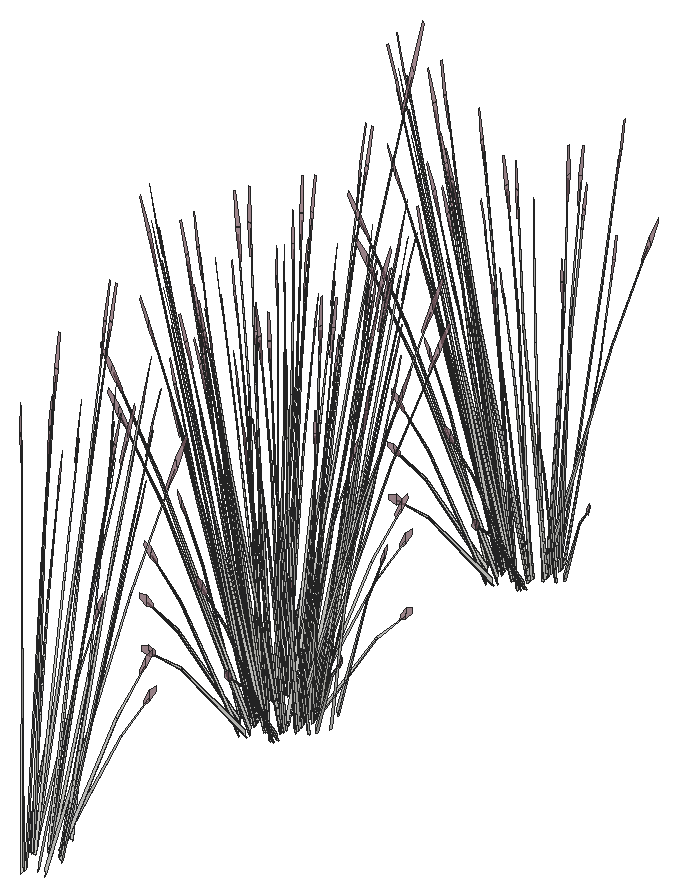
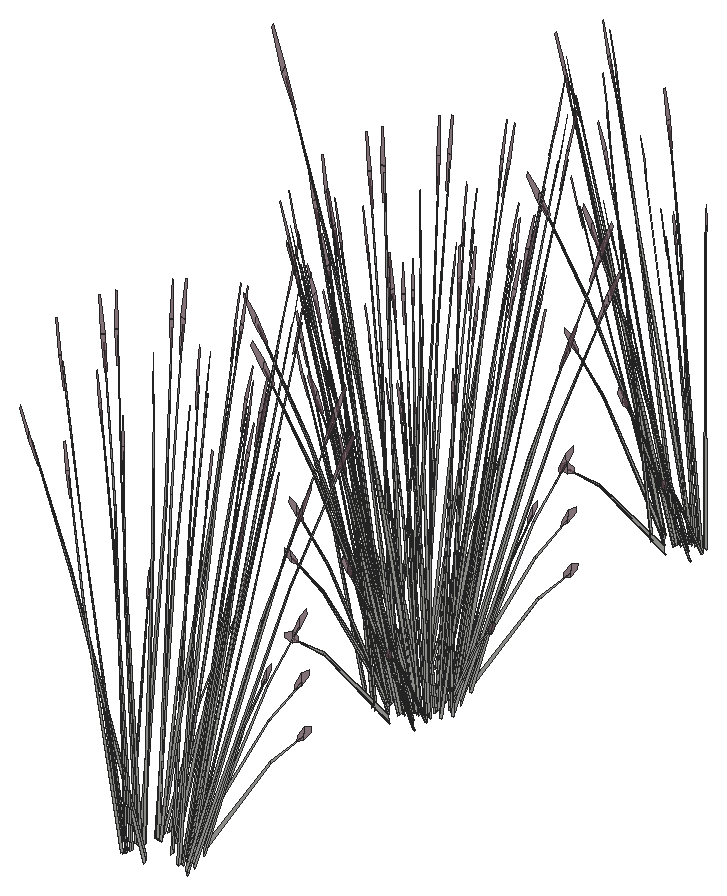
# SketchUp Ruby script. Lengths in inches.
U = 1.inch
M = Sketchup.active_model
def pt(a) = Geom::Point3d.new(a.map { |v| v * U })
def face(e, loops, mat)
  f = e.add_face(loops[0].map { |a| pt(a) })
  loops[1..].each { |l| e.add_face(l.map { |a| pt(a) }).erase! }
  f.material = f.back_material = mat if mat
  f
end
# faces: each face lists its corners as indices into pts; further lists are holes
def faces(e, pts, list, mat = nil) = list.each { |f| face(e, (f[0].is_a?(Array) ? f : [f]).map { |l| l.map { |i| pts[i] } }, mat) }
# xy, xz, yz: faces in a plane at the given z, y or x. An outline is a flat list of corners, or four numbers for a rectangle; further outlines are holes
def ring(l) = l.size == 4 ? [[l[0], l[1]], [l[2], l[1]], [l[2], l[3]], [l[0], l[3]]] : l.each_slice(2).to_a
def flat(e, list, mat, &to3) = list.each { |f| face(e, (f[0].is_a?(Array) ? f : [f]).map { |l| ring(l).map { |u, v| to3.(u, v) } }, mat) }
def xy(e, z, list, mat = nil) = flat(e, list, mat) { |x, y| [x, y, z] }
def xz(e, y, list, mat = nil) = flat(e, list, mat) { |x, z| [x, y, z] }
def yz(e, x, list, mat = nil) = flat(e, list, mat) { |y, z| [x, y, z] }
def lines(e, pts, list) = list.each { |a, b| e.add_line(pt(pts[a]), pt(pts[b])) }
# prism: a flat outline (further loops are holes) pulled along v
def prism(e, loops, v, mat = nil)
  f = face(e, loops, mat); d = Geom::Vector3d.new(v.map { |x| x * U })
  f.pushpull(f.normal.samedirection?(d) ? d.length : -d.length)
end
def box(e, o, s, mat = nil) = prism(e, [[o, [o[0] + s[0], o[1], o[2]], [o[0] + s[0], o[1] + s[1], o[2]], [o[0], o[1] + s[1], o[2]]]], [0, 0, s[2]], mat)
def at(x, y, z, deg = 0) = Geom::Transformation.translation(pt([x, y, z])) * Geom::Transformation.rotation(ORIGIN, Z_AXIS, deg.degrees)
def axes(o, x, y, z) = Geom::Transformation.new([*x, 0, *y, 0, *z, 0, *pt(o).to_a, 1])
def part(name) = M.definitions.add(name)
# library, detail: a bought-in or finely detailed component or shape, given as its bounding box
def library(name, o, s) = part(name).tap { |d| box(d.entities, o, s) }
def detail(e, o, s) = box(e.add_group.entities, o, s)
def put(e, d, t, mat = nil) = e.add_instance(d, t).tap { |i| i.material = mat if mat }
def group(e, t, mat = nil) = e.add_group.tap { |g| g.transformation = t; g.material = mat if mat }.entities
root = M.entities
M.materials.add("LightPink_Translucent").color = [144, 107, 117]
M.materials["LightPink_Translucent"].alpha = 0.75
c1 = part("blade")
p = [[2.15,0.21,22],[0,0.17,0],[0.09,0.45,0],[2.18,0.31,22],[2.29,0.31,22],[0.38,0.45,0],
  [2.48,0.24,33],[2.49,0.24,33],[2.48,0.22,33]]
faces(c1.entities,p,[[0,1,2,3],[4,5,2,3],[6,3,4,7],[8,0,3,6]])
c2 = part("seeds")
p = [[0.3,-0.1,1.38],[-0.01,-0.03,1.59],[-0.01,-0.03,0.03],[0.14,-0.07,-0.07],[0.29,-0.03,3],[0.15,0.01,3.11]]
faces(c2.entities,p,[[0,1,2,3],[1,0,4,5]],"LightPink_Translucent")
c3 = part("blade with seeds")
put(c3.entities,c1,at(0,0,0))
put(c3.entities,c2,axes([2.4,0.25,30.99],[1.5799,-0.05474,1.17369],[-0.12525,1.92788,0.29478],[-0.07173,-0.02425,1.56792]))
put(root,c3,axes([432.97,46.57,2.33],[0.22423,-0.47232,-0.10458],[0.32472,0.27211,-0.58045],[0.11288,0.13344,0.88199]))
put(root,c3,axes([431.35,44.86,1.33],[0.09398,-0.16955,1.47384],[0.23731,0.45764,0.11917],[-0.16276,0.20841,0.63005]))
put(root,c3,axes([431.49,45.93,2.34],[0.2546,-0.29052,0.30456],[0.24101,0.33173,-0.39319],[-0.03667,0.16855,0.75234]))
put(root,c3,axes([432.68,46.96,2.05],[0.00111,-0.06681,1.5255],[0.32247,-0.29474,-0.14414],[0.11201,0.1052,0.26996]))
put(root,c3,axes([431.26,46.2,2.07],[-0.30922,-0.02571,0.0553],[0.00848,-0.38824,0.43534],[-0.03236,0.14872,0.66383]))
put(root,c3,axes([431.36,46.23,2.07],[-0.26795,-0.37649,0.41282],[0.28456,-0.3247,0.34039],[-0.04943,0.17664,0.85423]))
put(root,c3,axes([432.21,46.41,2.34],[0.11344,-0.42434,0.30456],[0.33096,0.12377,-0.39319],[0.03035,0.17085,0.75234]))
put(root,c3,axes([433.05,46.74,2.07],[-0.17102,0.35053,0.0553],[-0.24354,-0.20408,0.43534],[0.07874,0.11238,0.66383]))
put(root,c3,axes([432.65,47.93,2.86],[0.26003,-0.31656,-0.05579],[0.23826,0.3467,-0.25298],[0.01677,0.09824,0.83441]))
put(root,c3,axes([433.125,46.65,2.07],[-0.37426,0.12663,0.41282],[-0.06495,-0.49674,0.34039],[0.08802,0.1464,0.85423]))
put(root,c3,axes([431.28,45.28,1.33],[0.07006,-0.18966,1.47384],[0.29392,0.3925,0.11917],[-0.13259,0.24463,0.63005]))
put(root,c3,axes([432.1,46.8,2.07],[-0.27727,0.18753,0.0553],[-0.13571,-0.34197,0.43534],[0.02678,0.15075,0.66383]))
put(root,c3,axes([430.48,46.26,2.05],[-0.00935,0.1092,1.50452],[0.26544,0.37987,-0.23794],[-0.06949,0.17964,0.12066]))
put(root,c3,axes([431.33,46.01,2.64],[0.41355,0.02734,-0.11608],[-0.0113,0.51765,-0.6443],[-0.02873,0.19937,0.97901]))
put(root,c3,axes([432.09,46.59,2.33],[0.36822,-0.25691,-0.10458],[0.18095,0.45596,-0.58045],[0.04858,0.19215,0.88199]))
put(root,c3,axes([432.2,46.76,2.35],[-0.37078,-0.14426,0.45823],[0.12679,-0.47426,0.37783],[0.02228,0.18651,0.9482]))
put(root,c3,axes([432.62,45.59,1.33],[-0.08601,-0.17716,1.47384],[0.39746,-0.14915,0.11917],[0.08983,0.27813,0.63005]))
put(root,c3,axes([430.45,47.38,2.05],[0.04269,-0.03331,1.5255],[0.35284,0.2216,-0.14414],[-0.00829,0.1845,0.26996]))
put(root,c3,axes([431.92,45.68,1.33],[-0.00921,-0.21179,1.47384],[0.39917,0.1405,0.11917],[-0.02469,0.30182,0.63005]))
put(root,c3,axes([432.01,47.61,2.05],[0.0477,0.08886,1.50452],[0.38493,0.03491,-0.23794],[0.03871,0.19596,0.12066]))
put(root,c3,axes([431.68,66.12,1.33],[0.08601,0.17716,1.47384],[-0.39746,0.14915,0.11917],[-0.08983,-0.27813,0.63005]))
put(root,c3,axes([432.33,64.95,2.05],[-0.05755,-0.07737,1.50452],[-0.38409,0.04905,-0.23794],[-0.0613,-0.18505,0.12066]))
put(root,c3,axes([434.06,65.89,2.05],[-0.00363,-0.10982,1.50452],[-0.30678,-0.3174,-0.23794],[0.04743,-0.1924,0.12066]))
put(root,c3,axes([433.02,66.43,1.33],[-0.07006,0.18966,1.47384],[-0.29392,-0.3925,0.11917],[0.13259,-0.24463,0.63005]))
put(root,c3,axes([433.98,65.5,2.05],[-0.03821,0.04215,1.5255],[-0.37441,-0.1422,-0.14414],[-0.01355,-0.18393,0.26996]))
put(root,c3,axes([431.9375,64.69,2.05],[-0.00702,0.06614,1.5255],[-0.34622,0.24004,-0.14414],[-0.10188,-0.1227,0.26996]))
put(root,c3,axes([431.86,65.87,2.38],[0.41917,-0.14183,0.46236],[0.07275,0.55635,0.38124],[-0.09858,-0.16397,0.95674]))
put(root,c3,axes([432.81,65.97,2.07],[0.37078,0.14426,0.41282],[-0.12679,0.47426,0.34039],[-0.02228,-0.18651,0.85423]))
put(root,c3,axes([432.92,66.14,2.33],[-0.36822,0.25691,-0.10458],[-0.18095,-0.45596,-0.58045],[-0.04858,-0.19215,0.88199]))
put(root,c3,axes([433.68,66.72,2.33],[-0.41355,-0.02734,-0.10458],[0.0113,-0.51765,-0.58045],[0.02873,-0.19937,0.88199]))
put(root,c3,axes([432.91,65.93,2.07],[0.27727,-0.18753,0.0553],[0.13571,0.34197,0.43534],[-0.02678,-0.15075,0.66383]))
put(root,c3,axes([431.96,65.99,2.07],[0.17102,-0.35053,0.0553],[0.24354,0.20408,0.43534],[-0.07874,-0.11238,0.66383]))
put(root,c3,axes([431.1,66.67,1.33],[0.13977,0.09507,1.47384],[-0.28925,0.39884,0.11917],[-0.18028,-0.17992,0.63005]))
put(root,c3,axes([432.81,66.32,2.34],[-0.11344,0.42434,0.30456],[-0.33096,-0.12377,-0.39319],[-0.03035,-0.17085,0.75234]))
put(root,c3,axes([433.65,66.5,2.07],[0.26795,0.37649,0.41282],[-0.28456,0.3247,0.34039],[0.04943,-0.17664,0.85423]))
put(root,c3,axes([432.04,65.95,2.67],[-0.25113,0.52899,-0.11713],[-0.36369,-0.30476,-0.65011],[-0.12642,-0.14945,0.98783]))
put(root,c3,axes([433.75,66.53,2.07],[0.30922,0.02571,0.0553],[-0.00848,0.38824,0.43534],[0.03236,-0.14872,0.66383]))
put(root,c3,axes([433.52,66.8,2.34],[-0.2546,0.29052,0.30456],[-0.24101,-0.33173,-0.39319],[0.03667,-0.16855,0.75234]))
put(root,c3,axes([431.07,65.8,2.05],[-0.08096,-0.00389,1.50452],[-0.25776,0.38949,-0.23794],[-0.13753,-0.07958,0.12066]))
put(root,c3,axes([434.13,67.73,2.33],[-0.34807,-0.30426,-0.10458],[0.20053,-0.44063,-0.58045],[0.09834,-0.15317,0.88199]))
put(root,c3,axes([432.01,66.39,2.34],[0.05812,0.44446,0.30456],[-0.33222,0.11736,-0.39319],[-0.08923,-0.12737,0.75234]))
put(root,c3,axes([431.01,66.68,2.38],[0.31075,-0.40722,0.46236],[0.268,0.43246,0.38124],[-0.14579,-0.07512,0.95674]))
put(root,c3,axes([434.99,67.6,2.05],[-0.04915,-0.00419,1.5255],[-0.20409,-0.44904,-0.14414],[0.08196,-0.14765,0.26996]))
put(root,c3,axes([431.16,66.68,2.07],[0.01895,-0.4196,0.0553],[0.28611,0.0115,0.43534],[-0.1096,-0.04391,0.66383]))
put(root,c3,axes([433.96,67.69,2.34],[-0.32754,0.07886,0.30456],[-0.08649,-0.45081,-0.39319],[0.09386,-0.12109,0.75234]))
put(root,c3,axes([434.26,67.62,2.07],[0.25832,0.23207,0.0553],[-0.1504,0.33047,0.43534],[0.08282,-0.10684,0.66383]))
put(root,c3,axes([434.1875,67.52,2.07],[0.09332,0.50785,0.41282],[-0.36608,0.08814,0.34039],[0.10789,-0.11944,0.85423]))
put(root,c3,axes([435.17,68.14,2.05],[0.05222,-0.08405,1.50452],[-0.06683,-0.51557,-0.23794],[0.13101,-0.09775,0.12066]))
put(root,c3,axes([430.76,66.13,2.05],[0.0279,0.05507,1.5255],[-0.13448,0.49501,-0.14414],[-0.1362,0.00358,0.26996]))
put(root,c3,axes([431.35,66.99,2.34],[0.2141,0.34548,0.30456],[-0.24447,0.32704,-0.39319],[-0.12421,-0.04976,0.75234]))
put(root,c3,axes([431.29,66.77,2.33],[-0.02015,0.56117,-0.10458],[-0.38148,-0.01534,-0.58045],[-0.14692,-0.03898,0.88199]))
put(root,c3,axes([434.15,68.92,2.33],[-0.18933,-0.49965,-0.10458],[0.33602,-0.24554,-0.58045],[0.1416,-0.06592,0.88199]))
put(root,c3,axes([430.81,67.54,1.33],[0.15608,-0.0125,1.47384],[-0.10354,0.54165,0.11917],[-0.22242,-0.0335,0.63005]))
put(root,c3,axes([434.01,68.77,2.34],[-0.31272,-0.15393,0.30456],[0.09121,-0.44909,-0.39319],[0.1259,-0.04118,0.75234]))
put(root,c3,axes([430.74,67.95,2.07],[0.10631,-0.50312,0.41282],[0.34951,0.17204,0.34039],[-0.13745,0.03024,0.85423]))
put(root,c3,axes([430.71,67.82,2.07],[-0.1382,-0.37624,0.0553],[0.25202,-0.18416,0.43534],[-0.11109,0.03633,0.66383]))
put(root,c3,axes([433.49,68.17,1.33],[-0.15608,0.0125,1.47384],[0.10354,-0.54165,0.11917],[0.22242,0.0335,0.63005]))
put(root,c3,axes([434.3,68.91,2.07],[0.1382,0.37624,0.0553],[-0.25202,0.18416,0.43534],[0.11109,-0.03633,0.66383]))
put(root,c3,axes([434.27,68.78,2.07],[-0.10631,0.50312,0.41282],[-0.34951,-0.17204,0.34039],[0.13745,-0.03024,0.85423]))
put(root,c3,axes([431,67.96,2.34],[0.31272,0.15393,0.30456],[-0.09121,0.44909,-0.39319],[-0.1259,0.04118,0.75234]))
put(root,c3,axes([434.9,70.41,2.05],[-0.03403,-0.04831,1.5255],[0.07443,-0.51782,-0.14414],[0.13402,-0.03308,0.26996]))
put(root,c3,axes([430.47,68.31,2.05],[-0.06145,0.07164,1.50452],[0.00523,0.52344,-0.23794],[-0.14085,0.06807,0.12066]))
put(root,c3,axes([430.87,67.81,2.33],[0.18933,0.49965,-0.10458],[-0.33602,0.24554,-0.58045],[-0.1416,0.06592,0.88199]))
put(root,c3,axes([434.6,69.97,1.38],[-0.07202,-0.46385,-0.03003],[0.3404,-0.10664,-0.13615],[0.07108,0.02941,0.44908]))
put(root,c3,axes([433.72,69.96,2.33],[0.02015,-0.56117,-0.10458],[0.38148,0.01534,-0.58045],[0.14692,0.03898,0.88199]))
put(root,c3,axes([433.66,69.74,2.34],[-0.2141,-0.34548,0.30456],[0.24447,-0.32704,-0.39319],[0.12421,0.04976,0.75234]))
put(root,c3,axes([434.05,69.625,2.05],[0.08072,-0.00933,1.50452],[0.22141,-0.42869,-0.23794],[0.14358,0.05659,0.12066]))
put(root,c3,axes([430.82,69.2,2.07],[-0.09332,-0.50785,0.41282],[0.36608,-0.08814,0.34039],[-0.10789,0.11944,0.85423]))
put(root,c3,axes([430.75,69.11,2.07],[-0.25832,-0.23207,0.0553],[0.1504,-0.33047,0.43534],[-0.08282,0.10684,0.66383]))
put(root,c3,axes([430.87,68.49,1.33],[0.13056,-0.11672,1.47384],[0.10992,0.53933,0.11917],[-0.20497,0.12189,0.63005]))
put(root,c3,axes([431.05,69.04,2.34],[0.32754,-0.07886,0.30456],[0.08649,0.45081,-0.39319],[-0.09386,0.12109,0.75234]))
put(root,c3,axes([429.79,68.83,2.05],[0.04802,0.0148,1.5255],[0.14856,0.48754,-0.14414],[-0.0983,0.12796,0.26996]))
put(root,c3,axes([433.86,70.05,2.07],[-0.01895,0.4196,0.0553],[-0.28611,-0.0115,0.43534],[0.1096,0.04391,0.66383]))
put(root,c3,axes([433.88,69.92,2.07],[-0.27746,0.36359,0.41282],[-0.23929,-0.38612,0.34039],[0.13017,0.06707,0.85423]))
put(root,c3,axes([430.31,70.32,2.86],[0.33205,0.14729,-0.05579],[-0.10214,0.45334,-0.25298],[-0.05431,0.06883,0.83441]))
put(root,c3,axes([433,70.34,2.34],[-0.05812,-0.44446,0.30456],[0.33222,-0.11736,-0.39319],[0.08923,0.12737,0.75234]))
put(root,c3,axes([433.2,69.04,1.33],[-0.13977,-0.09507,1.47384],[0.28925,-0.39884,0.11917],[0.18028,0.17992,0.63005]))
put(root,c3,axes([433.22,67.78,1.85],[-0.32515,-0.2867,1.18923],[0.34333,-0.44639,0.51312],[0.10491,0.26901,1.1495]))
put(root,c3,axes([430.88,68.99,2.33],[0.34807,0.30426,-0.10458],[-0.20053,0.44063,-0.58045],[-0.09834,0.15317,0.88199]))
put(root,c3,axes([432.97,70.57,2.33],[0.22423,-0.47232,-0.10458],[0.32472,0.27211,-0.58045],[0.11288,0.13344,0.88199]))
put(root,c3,axes([431.35,68.86,1.33],[0.09398,-0.16955,1.47384],[0.23731,0.45764,0.11917],[-0.16276,0.20841,0.63005]))
put(root,c3,axes([431.49,69.93,2.34],[0.2546,-0.29052,0.30456],[0.24101,0.33173,-0.39319],[-0.03667,0.16855,0.75234]))
put(root,c3,axes([432.68,70.96,2.05],[0.00111,-0.06681,1.5255],[0.32247,-0.29474,-0.14414],[0.11201,0.1052,0.26996]))
put(root,c3,axes([431.26,70.2,2.07],[-0.30922,-0.02571,0.0553],[0.00848,-0.38824,0.43534],[-0.03236,0.14872,0.66383]))
put(root,c3,axes([431.36,70.23,2.07],[-0.26795,-0.37649,0.41282],[0.28456,-0.3247,0.34039],[-0.04943,0.17664,0.85423]))
put(root,c3,axes([432.21,70.41,2.34],[0.11344,-0.42434,0.30456],[0.33096,0.12377,-0.39319],[0.03035,0.17085,0.75234]))
put(root,c3,axes([433.05,70.74,2.07],[-0.17102,0.35053,0.0553],[-0.24354,-0.20408,0.43534],[0.07874,0.11238,0.66383]))
put(root,c3,axes([432.65,71.93,2.86],[0.26003,-0.31656,-0.05579],[0.23826,0.3467,-0.25298],[0.01677,0.09824,0.83441]))
put(root,c3,axes([433.125,70.65,2.07],[-0.37426,0.12663,0.41282],[-0.06495,-0.49674,0.34039],[0.08802,0.1464,0.85423]))
put(root,c3,axes([431.28,69.28,1.33],[0.07006,-0.18966,1.47384],[0.29392,0.3925,0.11917],[-0.13259,0.24463,0.63005]))
put(root,c3,axes([432.1,70.8,2.07],[-0.27727,0.18753,0.0553],[-0.13571,-0.34197,0.43534],[0.02678,0.15075,0.66383]))
put(root,c3,axes([430.48,70.26,2.05],[-0.00935,0.1092,1.50452],[0.26544,0.37987,-0.23794],[-0.06949,0.17964,0.12066]))
put(root,c3,axes([431.33,70.01,2.64],[0.41355,0.02734,-0.11608],[-0.0113,0.51765,-0.6443],[-0.02873,0.19937,0.97901]))
put(root,c3,axes([432.09,70.59,2.33],[0.36822,-0.25691,-0.10458],[0.18095,0.45596,-0.58045],[0.04858,0.19215,0.88199]))
put(root,c3,axes([432.2,70.76,2.35],[-0.37078,-0.14426,0.45823],[0.12679,-0.47426,0.37783],[0.02228,0.18651,0.9482]))
put(root,c3,axes([432.62,69.59,1.33],[-0.08601,-0.17716,1.47384],[0.39746,-0.14915,0.11917],[0.08983,0.27813,0.63005]))
put(root,c3,axes([430.45,71.38,2.05],[0.04269,-0.03331,1.5255],[0.35284,0.2216,-0.14414],[-0.00829,0.1845,0.26996]))
put(root,c3,axes([431.92,69.68,1.33],[-0.00921,-0.21179,1.47384],[0.39917,0.1405,0.11917],[-0.02469,0.30182,0.63005]))
put(root,c3,axes([432.01,71.61,2.05],[0.0477,0.08886,1.50452],[0.38493,0.03491,-0.23794],[0.03871,0.19596,0.12066]))
put(root,c3,axes([431.68,89.33,1.33],[0.08601,0.17716,1.47384],[-0.39746,0.14915,0.11917],[-0.08983,-0.27813,0.63005]))
put(root,c3,axes([432.33,88.15,2.05],[-0.05755,-0.07737,1.50452],[-0.38409,0.04905,-0.23794],[-0.0613,-0.18505,0.12066]))
put(root,c3,axes([434.06,89.1,2.05],[-0.00363,-0.10982,1.50452],[-0.30678,-0.3174,-0.23794],[0.04743,-0.1924,0.12066]))
put(root,c3,axes([433.02,89.64,1.33],[-0.07006,0.18966,1.47384],[-0.29392,-0.3925,0.11917],[0.13259,-0.24463,0.63005]))
put(root,c3,axes([433.98,88.71,2.05],[-0.03821,0.04215,1.5255],[-0.37441,-0.1422,-0.14414],[-0.01355,-0.18393,0.26996]))
put(root,c3,axes([431.9375,87.9,2.05],[-0.00702,0.06614,1.5255],[-0.34622,0.24004,-0.14414],[-0.10188,-0.1227,0.26996]))
put(root,c3,axes([431.86,89.08,2.38],[0.41917,-0.14183,0.46236],[0.07275,0.55635,0.38124],[-0.09858,-0.16397,0.95674]))
put(root,c3,axes([432.81,89.18,2.07],[0.37078,0.14426,0.41282],[-0.12679,0.47426,0.34039],[-0.02228,-0.18651,0.85423]))
put(root,c3,axes([432.92,89.35,2.33],[-0.36822,0.25691,-0.10458],[-0.18095,-0.45596,-0.58045],[-0.04858,-0.19215,0.88199]))
put(root,c3,axes([433.68,89.93,2.33],[-0.41355,-0.02734,-0.10458],[0.0113,-0.51765,-0.58045],[0.02873,-0.19937,0.88199]))
put(root,c3,axes([432.91,89.14,2.07],[0.27727,-0.18753,0.0553],[0.13571,0.34197,0.43534],[-0.02678,-0.15075,0.66383]))
put(root,c3,axes([431.96,89.2,2.07],[0.17102,-0.35053,0.0553],[0.24354,0.20408,0.43534],[-0.07874,-0.11238,0.66383]))
put(root,c3,axes([431.1,89.88,1.33],[0.13977,0.09507,1.47384],[-0.28925,0.39884,0.11917],[-0.18028,-0.17992,0.63005]))
put(root,c3,axes([432.81,89.53,2.34],[-0.11344,0.42434,0.30456],[-0.33096,-0.12377,-0.39319],[-0.03035,-0.17085,0.75234]))
put(root,c3,axes([433.65,89.71,2.07],[0.26795,0.37649,0.41282],[-0.28456,0.3247,0.34039],[0.04943,-0.17664,0.85423]))
put(root,c3,axes([432.04,89.16,2.67],[-0.25113,0.52899,-0.11713],[-0.36369,-0.30476,-0.65011],[-0.12642,-0.14945,0.98783]))
put(root,c3,axes([433.75,89.74,2.07],[0.30922,0.02571,0.0553],[-0.00848,0.38824,0.43534],[0.03236,-0.14872,0.66383]))
put(root,c3,axes([433.52,90.01,2.34],[-0.2546,0.29052,0.30456],[-0.24101,-0.33173,-0.39319],[0.03667,-0.16855,0.75234]))
put(root,c3,axes([431.07,89.01,2.05],[-0.08096,-0.00389,1.50452],[-0.25776,0.38949,-0.23794],[-0.13753,-0.07958,0.12066]))
put(root,c3,axes([434.13,90.94,2.33],[-0.34807,-0.30426,-0.10458],[0.20053,-0.44063,-0.58045],[0.09834,-0.15317,0.88199]))
put(root,c3,axes([432.01,89.6,2.34],[0.05812,0.44446,0.30456],[-0.33222,0.11736,-0.39319],[-0.08923,-0.12737,0.75234]))
put(root,c3,axes([431.01,89.89,2.38],[0.31075,-0.40722,0.46236],[0.268,0.43246,0.38124],[-0.14579,-0.07512,0.95674]))
put(root,c3,axes([434.99,90.8125,2.05],[-0.04915,-0.00419,1.5255],[-0.20409,-0.44904,-0.14414],[0.08196,-0.14765,0.26996]))
put(root,c3,axes([431.16,89.89,2.07],[0.01895,-0.4196,0.0553],[0.28611,0.0115,0.43534],[-0.1096,-0.04391,0.66383]))
put(root,c3,axes([433.96,90.9,2.34],[-0.32754,0.07886,0.30456],[-0.08649,-0.45081,-0.39319],[0.09386,-0.12109,0.75234]))
put(root,c3,axes([434.26,90.83,2.07],[0.25832,0.23207,0.0553],[-0.1504,0.33047,0.43534],[0.08282,-0.10684,0.66383]))
put(root,c3,axes([434.1875,90.73,2.07],[0.09332,0.50785,0.41282],[-0.36608,0.08814,0.34039],[0.10789,-0.11944,0.85423]))
put(root,c3,axes([435.17,91.35,2.05],[0.05222,-0.08405,1.50452],[-0.06683,-0.51557,-0.23794],[0.13101,-0.09775,0.12066]))
put(root,c3,axes([430.76,89.34,2.05],[0.0279,0.05507,1.5255],[-0.13448,0.49501,-0.14414],[-0.1362,0.00358,0.26996]))
put(root,c3,axes([431.35,90.2,2.34],[0.2141,0.34548,0.30456],[-0.24447,0.32704,-0.39319],[-0.12421,-0.04976,0.75234]))
put(root,c3,axes([431.29,89.98,2.33],[-0.02015,0.56117,-0.10458],[-0.38148,-0.01534,-0.58045],[-0.14692,-0.03898,0.88199]))
put(root,c3,axes([434.15,92.13,2.33],[-0.18933,-0.49965,-0.10458],[0.33602,-0.24554,-0.58045],[0.1416,-0.06592,0.88199]))
put(root,c3,axes([430.81,90.75,1.33],[0.15608,-0.0125,1.47384],[-0.10354,0.54165,0.11917],[-0.22242,-0.0335,0.63005]))
put(root,c3,axes([434.01,91.98,2.34],[-0.31272,-0.15393,0.30456],[0.09121,-0.44909,-0.39319],[0.1259,-0.04118,0.75234]))
put(root,c3,axes([430.74,91.16,2.07],[0.10631,-0.50312,0.41282],[0.34951,0.17204,0.34039],[-0.13745,0.03024,0.85423]))
put(root,c3,axes([430.71,91.03,2.07],[-0.1382,-0.37624,0.0553],[0.25202,-0.18416,0.43534],[-0.11109,0.03633,0.66383]))
put(root,c3,axes([433.49,91.375,1.33],[-0.15608,0.0125,1.47384],[0.10354,-0.54165,0.11917],[0.22242,0.0335,0.63005]))
put(root,c3,axes([434.3,92.12,2.07],[0.1382,0.37624,0.0553],[-0.25202,0.18416,0.43534],[0.11109,-0.03633,0.66383]))
put(root,c3,axes([434.27,91.99,2.07],[-0.10631,0.50312,0.41282],[-0.34951,-0.17204,0.34039],[0.13745,-0.03024,0.85423]))
put(root,c3,axes([431,91.17,2.34],[0.31272,0.15393,0.30456],[-0.09121,0.44909,-0.39319],[-0.1259,0.04118,0.75234]))
